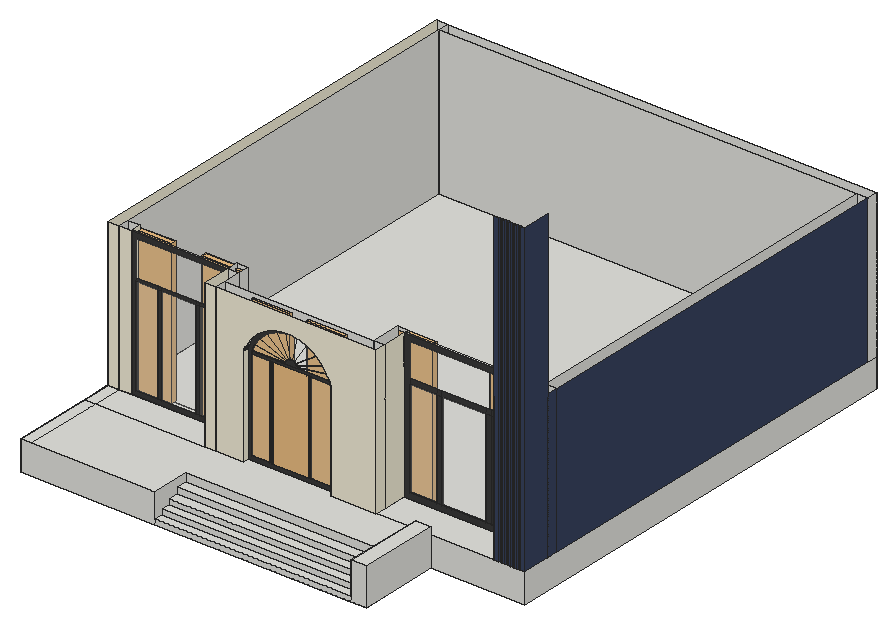
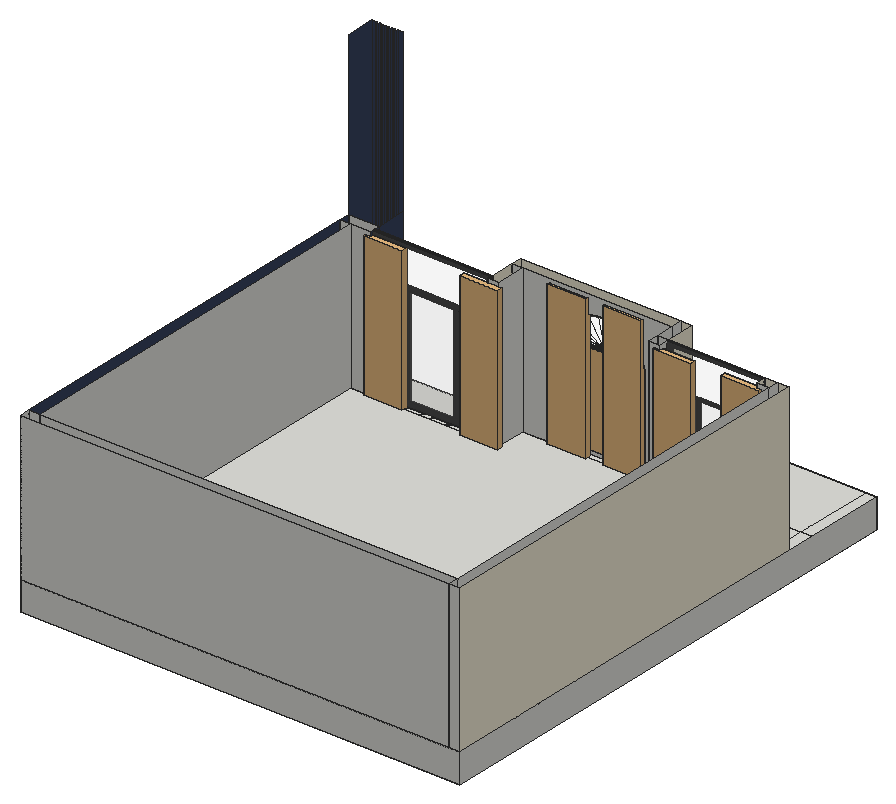
# SketchUp Ruby script. Lengths in inches.
U = 1.inch
M = Sketchup.active_model
def pt(a) = Geom::Point3d.new(a.map { |v| v * U })
def face(e, loops, mat)
  f = e.add_face(loops[0].map { |a| pt(a) })
  loops[1..].each { |l| e.add_face(l.map { |a| pt(a) }).erase! }
  f.material = f.back_material = mat if mat
  f
end
# faces: each face lists its corners as indices into pts; further lists are holes
def faces(e, pts, list, mat = nil) = list.each { |f| face(e, (f[0].is_a?(Array) ? f : [f]).map { |l| l.map { |i| pts[i] } }, mat) }
# xy, xz, yz: faces in a plane at the given z, y or x. An outline is a flat list of corners, or four numbers for a rectangle; further outlines are holes
def ring(l) = l.size == 4 ? [[l[0], l[1]], [l[2], l[1]], [l[2], l[3]], [l[0], l[3]]] : l.each_slice(2).to_a
def flat(e, list, mat, &to3) = list.each { |f| face(e, (f[0].is_a?(Array) ? f : [f]).map { |l| ring(l).map { |u, v| to3.(u, v) } }, mat) }
def xy(e, z, list, mat = nil) = flat(e, list, mat) { |x, y| [x, y, z] }
def xz(e, y, list, mat = nil) = flat(e, list, mat) { |x, z| [x, y, z] }
def yz(e, x, list, mat = nil) = flat(e, list, mat) { |y, z| [x, y, z] }
def lines(e, pts, list) = list.each { |a, b| e.add_line(pt(pts[a]), pt(pts[b])) }
# prism: a flat outline (further loops are holes) pulled along v
def prism(e, loops, v, mat = nil)
  f = face(e, loops, mat); d = Geom::Vector3d.new(v.map { |x| x * U })
  f.pushpull(f.normal.samedirection?(d) ? d.length : -d.length)
end
def box(e, o, s, mat = nil) = prism(e, [[o, [o[0] + s[0], o[1], o[2]], [o[0] + s[0], o[1] + s[1], o[2]], [o[0], o[1] + s[1], o[2]]]], [0, 0, s[2]], mat)
def at(x, y, z, deg = 0) = Geom::Transformation.translation(pt([x, y, z])) * Geom::Transformation.rotation(ORIGIN, Z_AXIS, deg.degrees)
def axes(o, x, y, z) = Geom::Transformation.new([*x, 0, *y, 0, *z, 0, *pt(o).to_a, 1])
def part(name) = M.definitions.add(name)
# library, detail: a bought-in or finely detailed component or shape, given as its bounding box
def library(name, o, s) = part(name).tap { |d| box(d.entities, o, s) }
def detail(e, o, s) = box(e.add_group.entities, o, s)
def put(e, d, t, mat = nil) = e.add_instance(d, t).tap { |i| i.material = mat if mat }
def group(e, t, mat = nil) = e.add_group.tap { |g| g.transformation = t; g.material = mat if mat }.entities
root = M.entities
M.materials.add("0360 AP 9644 Monsoon Midnight-N").color = [56, 67, 95]
M.materials.add("0905 AP 7844 MILD YELLOW").color = [242, 237, 215]
M.materials.add("Glass Clear 001").color = [246, 246, 246]
M.materials["Glass Clear 001"].alpha = 0.1
M.materials.add("[Color M07]").color = [58, 58, 58]
c1 = library("Curtains 004",[-15.59,-2.26,0],[31.18,4.52,116.91])
c2 = library("Door 243 053",[-21.6,-2.79,-0.07],[43.2,5.58,82.64])
xy(root,-24,[[24,0,24,425.9375,384,425.9375,384,65.9375,307.25,65.9375,307.25,0]])
xy(root,-19.71,[[134.39,0,294.77,6.625]])
xy(root,-15.42,[[134.39,6.625,294.77,14.1875]])
xy(root,-11.11,[[134.39,14.1875,294.77,22.4375]])
xy(root,-6.36,[[134.39,22.4375,294.77,31.5625]])
xy(root,0,[[24,0,33,65.9375],[33,0,134.39,0,134.39,31.5625,294.77,31.5625,294.77,65.9375,225.17,65.9375,225.17,70.4375,153.92,70.4375,153.92,65.9375,33,65.9375],[24,65.9375,33,89.9375],[33,65.9375,122.125,89.9375],[122.125,65.9375,153.92,65.9375,153.92,70.4375,225.17,70.4375,225.17,65.9375,262.5625,65.9375,262.5625,94.4375,358.89,94.4375,358.89,98.9375,253.5625,98.9375,253.5625,74.9375,131.125,74.9375,131.125,98.9375,43.05,98.9375,43.05,89.9375,122.125,89.9375],
  [122.125,65.9375,131.125,89.9375],[131.125,65.9375,153.92,74.9375],[225.17,65.9375,262.5625,74.9375],[262.5625,65.9375,358.89,94.4375],[358.89,65.9375,362.92,65.9375,362.92,66.75,365.27,66.75,365.27,65.9375,367.92,65.9375,367.92,66.75,370.27,66.75,370.27,65.9375,372.92,65.9375,372.92,66.75,375.27,66.75,375.27,65.9375,377.92,65.9375,377.92,66.75,380.27,66.75,380.27,65.9375,384,65.9375,384,89.9375,358.89,89.9375],
  [362.92,65.9375,365.27,66.75],[367.92,65.9375,370.27,66.75],[372.92,65.9375,375.27,66.75],[377.92,65.9375,380.27,66.75],[153.92,70.4375,225.17,70.75],
  [131.125,74.9375,253.5625,74.9375,253.5625,98.9375,375,98.9375,375,416.9375,33,416.9375,33,98.9375,131.125,98.9375],[253.5625,74.9375,262.5625,98.9375],[24,89.9375,33,425.9375],[33,89.9375,43.05,98.9375],[43.05,89.9375,122.125,91.4375],
  [122.125,89.9375,131.125,98.9375],[358.89,89.9375,384,98.9375],[43.05,91.4375,122.125,98.9375],[262.5625,94.4375,358.89,96.5625],[262.5625,96.5625,358.89,98.9375],
  [375,98.9375,384,416.9375],[33,416.9375,384,425.9375]])
xy(root,3.38,[[172.1875,70.4375,174.05,70.75],[203.54,70.4375,205.49,70.75]])
xy(root,3.38,[[157.31,70.4375,172.1875,70.75],[174.05,70.4375,203.54,70.75],[205.49,70.4375,221.79,70.75]],"[Color M07]")
xy(root,3.74,[[46.79,89.9375,64.29,90.25],[67.49,89.9375,95.54,90.25],[98.74,89.9375,118.39,90.25]],"[Color M07]")
xy(root,4.37,[[266.94,94.4375,289.69,95.5],[293.7,94.4375,329.88,95.5],[334.04,94.4375,354.52,95.5]],"[Color M07]")
xy(root,6.4375,[[294.77,0,307.25,65.9375]])
xy(root,78.21,[[157.31,70.4375,172.1875,70.75],[174.05,70.4375,203.54,70.75],[205.49,70.4375,221.79,70.75]],"[Color M07]")
xy(root,84.36,[[46.79,89.9375,64.29,90.25],[67.49,89.9375,95.54,90.25],[98.74,89.9375,118.39,90.25]])
xy(root,84.51,[[266.94,94.4375,289.69,95.5],[293.7,94.4375,329.88,95.5],[334.04,94.4375,354.52,95.5]])
xz(root,0,[[24,-24,134.39,0],[134.39,-24,294.77,-19.71],[294.77,-24,307.25,6.4375]])
xz(root,6.625,[[134.39,-19.71,294.77,-15.42]])
xz(root,14.1875,[[134.39,-15.42,294.77,-11.11]])
xz(root,22.4375,[[134.39,-11.11,294.77,-6.36]])
xz(root,31.5625,[[134.39,-6.36,294.77,0]])
xz(root,65.9375,[[307.25,-24,384,0],[294.77,0,307.25,6.4375]])
xz(root,65.9375,[[358.89,0,362.92,252],[365.27,0,367.92,252],[370.27,0,372.92,252],[375.27,0,377.92,252],[380.27,0,384,252]],"0360 AP 9644 Monsoon Midnight-N")
xz(root,65.9375,[[122.125,0,131.125,120],[131.125,0,153.92,0,153.92,81.13,154.18,81.87,154.45,82.6,154.73,83.33,155.03,84.05,155.35,84.77,155.68,85.48,156.02,86.18,156.38,86.87,156.76,87.56,157.15,88.24,157.55,88.91,157.96,89.57,158.39,90.22,158.84,90.87,159.29,91.5,159.76,92.125,160.25,92.74,160.74,93.35,161.25,93.94,161.77,94.53,162.3,95.1,162.84,95.66,163.4,96.21,163.97,96.75,164.54,97.28,165.13,97.79,165.73,98.29,166.34,98.78,166.96,99.26,167.59,99.72,168.23,100.17,168.875,100.61,169.53,101.03,170.2,101.44,170.875,101.84,171.56,102.22,172.25,102.59,172.94,102.94,173.65,103.28,174.36,103.6,175.08,103.91,175.8,104.21,176.53,104.48,177.27,104.75,178.01,105,178.76,105.23,179.51,105.45,180.26,105.65,181.02,105.83,181.79,106,182.55,106.16,183.32,106.29,184.1,106.41,184.87,106.52,185.65,106.61,186.42,106.68,187.2,106.74,187.99,106.78,188.77,106.8,189.55,106.8125,190.49,106.8,191.42,106.77,192.36,106.71,193.29,106.625,194.23,106.52,195.16,106.39,196.08,106.24,197,106.06,197.92,105.87,198.83,105.65,199.74,105.4,200.64,105.14,201.53,104.85,202.42,104.54,203.29,104.21,204.16,103.85,205.02,103.48,205.87,103.08,206.71,102.66,207.54,102.22,208.36,101.76,209.16,101.28,209.96,100.78,210.74,100.26,211.51,99.72,212.26,99.16,213,98.59,213.73,97.99,214.4375,97.38,215.13,96.75,215.81,96.1,216.47,95.4375,217.12,94.76,217.75,94.06,218.36,93.35,218.95,92.62,219.52,91.88,220.08,91.12,220.62,90.35,221.13,89.57,221.63,88.77,222.11,87.97,222.57,87.15,223,86.32,223.42,85.48,223.8125,84.625,224.18,83.76,224.54,82.89,224.87,82.02,225.17,81.13,225.17,0,262.5625,0,262.5625,120,131.125,120]],"0905 AP 7844 MILD YELLOW")
xz(root,66.75,[[362.92,0,365.27,252],[367.92,0,370.27,252],[372.92,0,375.27,252],[377.92,0,380.27,252]],"0360 AP 9644 Monsoon Midnight-N")
xz(root,70.4375,[[[153.92,0,225.17,0,225.17,81.13,224.87,82.02,224.54,82.89,224.18,83.76,223.8125,84.625,223.42,85.48,223,86.32,222.57,87.15,222.11,87.97,221.63,88.77,221.13,89.57,220.62,90.35,220.08,91.12,219.52,91.88,218.95,92.62,218.36,93.35,217.75,94.06,217.12,94.76,216.47,95.4375,215.81,96.1,215.13,96.75,214.4375,97.38,213.73,97.99,213,98.59,212.26,99.16,211.51,99.72,210.74,100.26,209.96,100.78,209.16,101.28,208.36,101.76,207.54,102.22,206.71,102.66,205.87,103.08,205.02,103.48,204.16,103.85,203.29,104.21,202.42,104.54,201.53,104.85,200.64,105.14,199.74,105.4,198.83,105.65,197.92,105.87,197,106.06,196.08,106.24,195.16,106.39,194.23,106.52,193.29,106.625,192.36,106.71,191.42,106.77,190.49,106.8,189.55,106.8125,188.77,106.8,187.99,106.78,187.2,106.74,186.42,106.68,185.65,106.61,184.87,106.52,184.1,106.41,183.32,106.29,182.55,106.16,181.79,106,181.02,105.83,180.26,105.65,179.51,105.45,178.76,105.23,178.01,105,177.27,104.75,176.53,104.48,175.8,104.21,175.08,103.91,174.36,103.6,173.65,103.28,172.94,102.94,172.25,102.59,171.56,102.22,170.875,101.84,170.2,101.44,169.53,101.03,168.875,100.61,168.23,100.17,167.59,99.72,166.96,99.26,166.34,98.78,165.73,98.29,165.13,97.79,164.54,97.28,163.97,96.75,163.4,96.21,162.84,95.66,162.3,95.1,161.77,94.53,161.25,93.94,160.74,93.35,160.25,92.74,159.76,92.125,159.29,91.5,158.84,90.87,158.39,90.22,157.96,89.57,157.55,88.91,157.15,88.24,156.76,87.56,156.38,86.87,156.02,86.18,155.68,85.48,155.35,84.77,155.03,84.05,154.73,83.33,154.45,82.6,154.18,81.87,153.92,81.13],[157.31,3.38,157.31,80.5625,157.61,81.4,157.87,82.0625,158.15,82.72,158.43,83.37,158.73,84.01,159.05,84.65,159.375,85.28,159.71,85.91,160.07,86.53,160.43,87.14,160.8125,87.74,161.2,88.33,161.6,88.92,162.02,89.5,162.45,90.07,162.89,90.625,163.34,91.18,163.8,91.72,164.27,92.25,164.76,92.77,165.25,93.28,165.76,93.78,166.27,94.27,166.8,94.75,167.33,95.22,167.88,95.68,168.43,96.12,169.57,96.98,170.15,97.39,170.74,97.78,171.34,98.17,171.94,98.54,172.56,98.9,173.18,99.25,174.44,99.91,175.08,100.21,175.73,100.51,176.38,100.79,177.04,101.06,177.71,101.31,178.375,101.55,179.05,101.78,179.73,101.99,180.41,102.18,181.1,102.37,181.79,102.54,182.49,102.69,183.18,102.83,183.88,102.96,184.59,103.07,185.29,103.16,186,103.24,186.71,103.31,187.42,103.36,188.125,103.4,188.84,103.42,189.54,103.43,190.4,103.42,191.26,103.39,192.11,103.33,192.96,103.26,193.81,103.16,194.65,103.04,195.49,102.91,196.33,102.75,197.17,102.57,198,102.37,198.82,102.15,199.64,101.9,200.45,101.64,201.26,101.36,202.06,101.06,202.85,100.73,203.63,100.39,204.4,100.03,205.16,99.65,205.92,99.25,206.66,98.83,207.4,98.4,208.12,97.94,208.83,97.47,209.53,96.98,210.21,96.47,210.89,95.94,211.55,95.4,212.19,94.85,212.83,94.27,213.44,93.68,214.05,93.08,214.63,92.46,215.2,91.82,215.76,91.18,216.3,90.51,216.82,89.84,217.33,89.15,217.82,88.45,218.29,87.74,218.74,87.02,219.17,86.28,219.59,85.54,219.99,84.78,220.36,84.01,220.72,83.24,221.0625,82.46,221.38,81.67,221.68,80.87,221.79,80.56,221.79,3.38]],[172.1875,3.38,174.05,78.21],[203.54,3.38,205.49,78.21],[157.31,78.21,221.79,78.21,221.79,80.56,195.3125,80.63,183.84,80.66,157.37,80.73,157.31,80.5625],[195.3125,80.63,194.98,81.38,194.8,81.78,194.43,82.28,194.06,82.79,193.51,83.29,193.12,83.63,192.03,84.26,191.98,84.28,190.84,84.65,190.49,84.69,189.59,84.79,188.68,84.69,188.34,84.66,187.3125,84.33,187.14,84.28,186.05,83.65,185.97,83.59,185.11,82.82,184.97,82.625,184.36,81.81,184.26,81.58,183.84,80.66]],"[Color M07]")
xz(root,70.75,[[[153.92,0,153.92,81.13,154.18,81.87,154.45,82.6,154.73,83.33,155.03,84.05,155.35,84.77,155.68,85.48,156.02,86.18,156.38,86.87,156.76,87.56,157.15,88.24,157.55,88.91,157.96,89.57,158.39,90.22,158.84,90.87,159.29,91.5,159.76,92.125,160.25,92.74,160.74,93.35,161.25,93.94,161.77,94.53,162.3,95.1,162.84,95.66,163.4,96.21,163.97,96.75,164.54,97.28,165.13,97.79,165.73,98.29,166.34,98.78,166.96,99.26,167.59,99.72,168.23,100.17,168.875,100.61,169.53,101.03,170.2,101.44,170.875,101.84,171.56,102.22,172.25,102.59,172.94,102.94,173.65,103.28,174.36,103.6,175.08,103.91,175.8,104.21,176.53,104.48,177.27,104.75,178.01,105,178.76,105.23,179.51,105.45,180.26,105.65,181.02,105.83,181.79,106,182.55,106.16,183.32,106.29,184.1,106.41,184.87,106.52,185.65,106.61,186.42,106.68,187.2,106.74,187.99,106.78,188.77,106.8,189.55,106.8125,190.49,106.8,191.42,106.77,192.36,106.71,193.29,106.625,194.23,106.52,195.16,106.39,196.08,106.24,197,106.06,197.92,105.87,198.83,105.65,199.74,105.4,200.64,105.14,201.53,104.85,202.42,104.54,203.29,104.21,204.16,103.85,205.02,103.48,205.87,103.08,206.71,102.66,207.54,102.22,208.36,101.76,209.16,101.28,209.96,100.78,210.74,100.26,211.51,99.72,212.26,99.16,213,98.59,213.73,97.99,214.4375,97.38,215.13,96.75,215.81,96.1,216.47,95.4375,217.12,94.76,217.75,94.06,218.36,93.35,218.95,92.62,219.52,91.88,220.08,91.12,220.62,90.35,221.13,89.57,221.63,88.77,222.11,87.97,222.57,87.15,223,86.32,223.42,85.48,223.8125,84.625,224.18,83.76,224.54,82.89,224.87,82.02,225.17,81.13,225.17,0],[157.31,3.38,221.79,3.38,221.79,80.56,221.68,80.87,221.38,81.67,221.0625,82.46,220.72,83.24,220.36,84.01,219.99,84.78,219.59,85.54,219.17,86.28,218.74,87.02,218.29,87.74,217.82,88.45,217.33,89.15,216.82,89.84,216.3,90.51,215.76,91.18,215.2,91.82,214.63,92.46,214.05,93.08,213.44,93.68,212.83,94.27,212.19,94.85,211.55,95.4,210.89,95.94,210.21,96.47,209.53,96.98,208.83,97.47,208.12,97.94,207.4,98.4,206.66,98.83,205.92,99.25,205.16,99.65,204.4,100.03,203.63,100.39,202.85,100.73,202.06,101.06,201.26,101.36,200.45,101.64,199.64,101.9,198.82,102.15,198,102.37,197.17,102.57,196.33,102.75,195.49,102.91,194.65,103.04,193.81,103.16,192.96,103.26,192.11,103.33,191.26,103.39,190.4,103.42,189.54,103.43,188.84,103.42,188.125,103.4,187.42,103.36,186.71,103.31,186,103.24,185.29,103.16,184.59,103.07,183.88,102.96,183.18,102.83,182.49,102.69,181.79,102.54,181.1,102.37,180.41,102.18,179.73,101.99,179.05,101.78,178.375,101.55,177.71,101.31,177.04,101.06,176.38,100.79,175.73,100.51,175.08,100.21,174.44,99.91,173.18,99.25,172.56,98.9,171.94,98.54,171.34,98.17,170.74,97.78,170.15,97.39,169.57,96.98,168.43,96.12,167.88,95.68,167.33,95.22,166.8,94.75,166.27,94.27,165.76,93.78,165.25,93.28,164.76,92.77,164.27,92.25,163.8,91.72,163.34,91.18,162.89,90.625,162.45,90.07,162.02,89.5,161.6,88.92,161.2,88.33,160.8125,87.74,160.43,87.14,160.07,86.53,159.71,85.91,159.375,85.28,159.05,84.65,158.73,84.01,158.43,83.37,158.15,82.72,157.87,82.0625,157.61,81.4,157.31,80.5625]]])
xz(root,70.75,[[157.31,3.38,172.1875,78.21],[205.49,3.38,221.79,78.21],[221.79,80.56,221.68,80.87,221.38,81.67,221.0625,82.46,220.72,83.24,220.36,84.01,219.99,84.78,194.98,81.38,195.3125,80.63],[183.84,80.66,184.26,81.58,159.71,85.91,159.375,85.28,159.05,84.65,158.73,84.01,158.43,83.37,158.15,82.72,157.87,82.0625,157.61,81.4,157.37,80.73],[194.98,81.38,219.99,84.78,219.59,85.54,219.17,86.28,218.74,87.02,218.29,87.74,217.82,88.45,217.33,89.15,216.82,89.84,194.43,82.28,194.8,81.78],
  [184.26,81.58,184.36,81.81,184.97,82.625,163.8,91.72,163.34,91.18,162.89,90.625,162.45,90.07,162.02,89.5,161.6,88.92,161.2,88.33,160.8125,87.74,160.43,87.14,160.07,86.53,159.71,85.91],[194.43,82.28,216.82,89.84,216.3,90.51,215.76,91.18,215.2,91.82,214.63,92.46,214.05,93.08,213.44,93.68,212.83,94.27,212.19,94.85,211.55,95.4,193.51,83.29,194.06,82.79],[184.97,82.625,185.11,82.82,185.97,83.59,169.57,96.98,168.43,96.12,167.88,95.68,167.33,95.22,166.8,94.75,166.27,94.27,165.76,93.78,165.25,93.28,164.76,92.77,164.27,92.25,163.8,91.72],[193.51,83.29,211.55,95.4,210.89,95.94,210.21,96.47,209.53,96.98,208.83,97.47,208.12,97.94,207.4,98.4,206.66,98.83,205.92,99.25,205.16,99.65,204.4,100.03,203.63,100.39,202.85,100.73,191.98,84.28,192.03,84.26,193.12,83.63],[185.97,83.59,186.05,83.65,187.14,84.28,187.3125,84.33,177.04,101.06,176.38,100.79,175.73,100.51,175.08,100.21,174.44,99.91,173.18,99.25,172.56,98.9,171.94,98.54,171.34,98.17,170.74,97.78,170.15,97.39,169.57,96.98],
  [191.98,84.28,202.85,100.73,202.06,101.06,201.26,101.36,200.45,101.64,199.64,101.9,198.82,102.15,198,102.37,197.17,102.57,196.33,102.75,195.49,102.91,194.65,103.04,190.49,84.69,190.84,84.65],[187.3125,84.33,188.34,84.66,188.68,84.69,184.59,103.07,183.88,102.96,183.18,102.83,182.49,102.69,181.79,102.54,181.1,102.37,180.41,102.18,179.73,101.99,179.05,101.78,178.375,101.55,177.71,101.31,177.04,101.06],[188.68,84.69,189.59,84.79,190.49,84.69,194.65,103.04,193.81,103.16,192.96,103.26,192.11,103.33,191.26,103.39,190.4,103.42,189.54,103.43,188.84,103.42,188.125,103.4,187.42,103.36,186.71,103.31,186,103.24,185.29,103.16,184.59,103.07]],"Glass Clear 001")
xz(root,74.9375,[[131.125,0,131.125,120,253.5625,120,253.5625,0,225.17,0,225.17,81.13,224.87,82.02,224.54,82.89,224.18,83.76,223.8125,84.625,223.42,85.48,223,86.32,222.57,87.15,222.11,87.97,221.63,88.77,221.13,89.57,220.62,90.35,220.08,91.12,219.52,91.88,218.95,92.62,218.36,93.35,217.75,94.06,217.12,94.76,216.47,95.4375,215.81,96.1,215.13,96.75,214.4375,97.38,213.73,97.99,213,98.59,212.26,99.16,211.51,99.72,210.74,100.26,209.96,100.78,209.16,101.28,208.36,101.76,207.54,102.22,206.71,102.66,205.87,103.08,205.02,103.48,204.16,103.85,203.29,104.21,202.42,104.54,201.53,104.85,200.64,105.14,199.74,105.4,198.83,105.65,197.92,105.87,197,106.06,196.08,106.24,195.16,106.39,194.23,106.52,193.29,106.625,192.36,106.71,191.42,106.77,190.49,106.8,189.55,106.8125,188.77,106.8,187.99,106.78,187.2,106.74,186.42,106.68,185.65,106.61,184.87,106.52,184.1,106.41,183.32,106.29,182.55,106.16,181.79,106,181.02,105.83,180.26,105.65,179.51,105.45,178.76,105.23,178.01,105,177.27,104.75,176.53,104.48,175.8,104.21,175.08,103.91,174.36,103.6,173.65,103.28,172.94,102.94,172.25,102.59,171.56,102.22,170.875,101.84,170.2,101.44,169.53,101.03,168.875,100.61,168.23,100.17,167.59,99.72,166.96,99.26,166.34,98.78,165.73,98.29,165.13,97.79,164.54,97.28,163.97,96.75,163.4,96.21,162.84,95.66,162.3,95.1,161.77,94.53,161.25,93.94,160.74,93.35,160.25,92.74,159.76,92.125,159.29,91.5,158.84,90.87,158.39,90.22,157.96,89.57,157.55,88.91,157.15,88.24,156.76,87.56,156.38,86.87,156.02,86.18,155.68,85.48,155.35,84.77,155.03,84.05,154.73,83.33,154.45,82.6,154.18,81.87,153.92,81.13,153.92,0],[253.5625,0,262.5625,120]])
xz(root,89.9375,[[122.125,0,131.125,120],[358.89,0,384,120]])
xz(root,89.9375,[[24,0,33,120],[33,0,43.05,120]],"0905 AP 7844 MILD YELLOW")
xz(root,89.9375,[[[43.05,0,122.125,120],[46.79,3.74,118.39,116.26]],[64.29,3.74,67.49,84.36],[95.54,3.74,98.74,84.36],[46.79,84.36,64.29,86.69],[64.29,84.36,67.49,86.69],
  [67.49,84.36,95.54,86.69],[95.54,84.36,98.74,86.69],[98.74,84.36,118.39,86.69]],"[Color M07]")
xz(root,90.25,[[46.79,3.74,64.29,84.36],[67.49,3.74,95.54,84.36],[98.74,3.74,118.39,84.36]],"Glass Clear 001")
xz(root,91.4375,[[43.05,0,122.125,120]],"Glass Clear 001")
xz(root,94.4375,[[[262.5625,0,358.89,120],[266.94,4.37,354.52,115.63]],[289.69,4.37,293.7,84.51],[329.88,4.37,334.04,84.51],[266.94,84.51,289.69,88.49],[289.69,84.51,293.7,88.49],
  [293.7,84.51,329.88,88.49],[329.88,84.51,334.04,88.49],[334.04,84.51,354.52,88.49]],"[Color M07]")
xz(root,95.5,[[266.94,4.37,289.69,84.51],[293.7,4.37,329.88,84.51],[334.04,4.37,354.52,84.51]],"Glass Clear 001")
xz(root,96.5625,[[262.5625,0,358.89,120]],"Glass Clear 001")
xz(root,98.9375,[[33,0,43.05,120],[122.125,0,131.125,120],[253.5625,0,262.5625,120],[358.89,0,375,120],[375,0,384,120]])
xz(root,416.9375,[[33,0,375,120],[375,0,384,120]])
xz(root,425.9375,[[24,-24,384,0],[24,0,33,120],[33,0,384,120]])
yz(root,24,[[0,-24,425.9375,0]])
yz(root,24,[[89.9375,0,425.9375,120]],"0905 AP 7844 MILD YELLOW")
yz(root,33,[[89.9375,0,98.9375,120],[98.9375,0,416.9375,120],[416.9375,0,425.9375,120]])
yz(root,43.05,[[91.4375,0,98.9375,120]],"0905 AP 7844 MILD YELLOW")
yz(root,43.05,[[89.9375,0,91.4375,120]],"[Color M07]")
yz(root,46.79,[[89.9375,3.74,90.25,84.36]],"[Color M07]")
yz(root,64.29,[[89.9375,3.74,90.25,84.36]],"[Color M07]")
yz(root,67.49,[[89.9375,3.74,90.25,84.36]],"[Color M07]")
yz(root,95.54,[[89.9375,3.74,90.25,84.36]],"[Color M07]")
yz(root,98.74,[[89.9375,3.74,90.25,84.36]],"[Color M07]")
yz(root,118.39,[[89.9375,3.74,90.25,84.36]],"[Color M07]")
yz(root,122.125,[[91.4375,0,98.9375,120]])
yz(root,122.125,[[65.9375,0,89.9375,120]],"0905 AP 7844 MILD YELLOW")
yz(root,122.125,[[89.9375,0,91.4375,120]],"[Color M07]")
yz(root,131.125,[[65.9375,0,74.9375,120],[74.9375,0,89.9375,120],[89.9375,0,98.9375,120]])
yz(root,134.39,[[0,-19.71,6.625,-19.71,6.625,-15.42,14.1875,-15.42,14.1875,-11.11,22.4375,-11.11,22.4375,-6.36,31.5625,-6.36,31.5625,0,0,0]])
yz(root,153.92,[[65.9375,0,70.4375,81.13],[70.75,0,74.9375,81.13]],"0905 AP 7844 MILD YELLOW")
yz(root,153.92,[[70.4375,0,70.75,81.13]],"[Color M07]")
yz(root,157.31,[[70.4375,78.21,70.75,80.5625]])
yz(root,157.31,[[70.4375,3.38,70.75,78.21]],"[Color M07]")
yz(root,172.1875,[[70.4375,3.38,70.75,78.21]],"[Color M07]")
yz(root,174.05,[[70.4375,3.38,70.75,78.21]],"[Color M07]")
yz(root,203.54,[[70.4375,3.38,70.75,78.21]],"[Color M07]")
yz(root,205.49,[[70.4375,3.38,70.75,78.21]],"[Color M07]")
yz(root,221.79,[[70.4375,78.21,70.75,80.56]])
yz(root,221.79,[[70.4375,3.38,70.75,78.21]],"[Color M07]")
yz(root,225.17,[[65.9375,0,70.4375,81.13],[70.75,0,74.9375,81.13]],"0905 AP 7844 MILD YELLOW")
yz(root,225.17,[[70.4375,0,70.75,81.13]],"[Color M07]")
yz(root,253.5625,[[74.9375,0,98.9375,120]])
yz(root,262.5625,[[65.9375,0,74.9375,120],[74.9375,0,94.4375,120],[96.5625,0,98.9375,120]],"0905 AP 7844 MILD YELLOW")
yz(root,262.5625,[[94.4375,0,96.5625,120]],"[Color M07]")
yz(root,266.94,[[94.4375,4.37,95.5,84.51]],"[Color M07]")
yz(root,289.69,[[94.4375,4.37,95.5,84.51]],"[Color M07]")
yz(root,293.7,[[94.4375,4.37,95.5,84.51]],"[Color M07]")
yz(root,294.77,[[0,-19.71,0,6.4375,65.9375,6.4375,65.9375,0,31.5625,0,31.5625,-6.36,22.4375,-6.36,22.4375,-11.11,14.1875,-11.11,14.1875,-15.42,6.625,-15.42,6.625,-19.71]])
yz(root,307.25,[[0,-24,65.9375,6.4375]])
yz(root,329.88,[[94.4375,4.37,95.5,84.51]],"[Color M07]")
yz(root,334.04,[[94.4375,4.37,95.5,84.51]],"[Color M07]")
yz(root,354.52,[[94.4375,4.37,95.5,84.51]],"[Color M07]")
yz(root,358.89,[[65.9375,0,89.9375,120],[89.9375,0,94.4375,120],[96.5625,0,98.9375,120]],"0360 AP 9644 Monsoon Midnight-N")
yz(root,358.89,[[94.4375,0,96.5625,120]],"[Color M07]")
yz(root,362.92,[[65.9375,0,66.75,252]],"0360 AP 9644 Monsoon Midnight-N")
yz(root,365.27,[[65.9375,0,66.75,252]],"0360 AP 9644 Monsoon Midnight-N")
yz(root,367.92,[[65.9375,0,66.75,252]],"0360 AP 9644 Monsoon Midnight-N")
yz(root,370.27,[[65.9375,0,66.75,252]],"0360 AP 9644 Monsoon Midnight-N")
yz(root,372.92,[[65.9375,0,66.75,252]],"0360 AP 9644 Monsoon Midnight-N")
yz(root,375,[[98.9375,0,416.9375,120]])
yz(root,375.27,[[65.9375,0,66.75,252]],"0360 AP 9644 Monsoon Midnight-N")
yz(root,377.92,[[65.9375,0,66.75,252]],"0360 AP 9644 Monsoon Midnight-N")
yz(root,380.27,[[65.9375,0,66.75,252]],"0360 AP 9644 Monsoon Midnight-N")
yz(root,384,[[65.9375,-24,425.9375,0],[416.9375,0,425.9375,120]])
yz(root,384,[[65.9375,0,89.9375,252],[89.9375,0,98.9375,120],[98.9375,0,416.9375,120]],"0360 AP 9644 Monsoon Midnight-N")
p = [[157.31,70.75,80.5625],[157.37,70.75,80.73],[157.37,70.4375,80.73],[157.31,70.4375,80.5625],[195.3125,70.75,80.63],[194.98,70.75,81.38],
  [194.98,70.4375,81.38],[195.3125,70.4375,80.63],[221.79,70.75,80.56],[221.79,70.4375,80.56],[221.68,70.75,80.87],[221.68,70.4375,80.87],
  [183.84,70.75,80.66],[183.84,70.4375,80.66],[157.61,70.75,81.4],[157.61,70.4375,81.4],[184.26,70.75,81.58],[184.26,70.4375,81.58],
  [221.38,70.75,81.67],[221.38,70.4375,81.67],[153.92,65.9375,81.13],[153.92,70.4375,81.13],[154.18,70.4375,81.87],[154.18,65.9375,81.87],
  [224.87,65.9375,82.02],[224.87,70.4375,82.02],[225.17,70.4375,81.13],[225.17,65.9375,81.13],[154.18,70.75,81.87],[153.92,70.75,81.13],
  [225.17,70.75,81.13],[224.87,70.75,82.02],[154.18,74.9375,81.87],[153.92,74.9375,81.13],[225.17,74.9375,81.13],[224.87,74.9375,82.02],
  [157.87,70.75,82.0625],[157.87,70.4375,82.0625],[194.8,70.75,81.78],[194.8,70.4375,81.78],[184.36,70.75,81.81],[184.36,70.4375,81.81],
  [221.0625,70.75,82.46],[221.0625,70.4375,82.46],[184.97,70.75,82.625],[184.97,70.4375,82.625],[194.43,70.75,82.28],[194.43,70.4375,82.28],
  [154.45,70.4375,82.6],[154.45,65.9375,82.6],[154.45,70.75,82.6],[154.45,74.9375,82.6],[224.54,65.9375,82.89],[224.54,70.4375,82.89],
  [224.54,70.75,82.89],[224.54,74.9375,82.89],[158.15,70.75,82.72],[158.15,70.4375,82.72],[194.06,70.75,82.79],[194.06,70.4375,82.79],
  [220.72,70.75,83.24],[220.72,70.4375,83.24],[154.73,70.4375,83.33],[154.73,65.9375,83.33],[154.73,70.75,83.33],[185.11,70.75,82.82],
  [185.11,70.4375,82.82],[154.73,74.9375,83.33],[158.43,70.75,83.37],[158.43,70.4375,83.37],[185.97,70.75,83.59],[185.97,70.4375,83.59],
  [193.51,70.75,83.29],[193.51,70.4375,83.29],[224.18,65.9375,83.76],[224.18,70.4375,83.76],[224.18,70.75,83.76],[224.18,74.9375,83.76],
  [220.36,70.75,84.01],[220.36,70.4375,84.01],[155.03,70.4375,84.05],[155.03,65.9375,84.05],[155.03,70.75,84.05],[193.12,70.75,83.63],
  [193.12,70.4375,83.63],[155.03,74.9375,84.05],[158.73,70.75,84.01],[158.73,70.4375,84.01],[186.05,70.75,83.65],[186.05,70.4375,83.65],
  [192.03,70.75,84.26],[192.03,70.4375,84.26],[187.14,70.75,84.28],[187.14,70.4375,84.28],[223.8125,65.9375,84.625],[223.8125,70.4375,84.625],
  [223.8125,70.75,84.625],[223.8125,74.9375,84.625],[159.05,70.75,84.65],[159.05,70.4375,84.65],[219.99,70.75,84.78],[219.99,70.4375,84.78],
  [155.35,70.4375,84.77],[155.35,65.9375,84.77],[155.35,70.75,84.77],[155.35,74.9375,84.77],[187.3125,70.75,84.33],[187.3125,70.4375,84.33],
  [188.34,70.75,84.66],[188.34,70.4375,84.66],[191.98,70.75,84.28],[190.84,70.75,84.65],[190.84,70.4375,84.65],[191.98,70.4375,84.28],
  [223.42,65.9375,85.48],[223.42,70.4375,85.48],[223.42,70.75,85.48],[223.42,74.9375,85.48],[159.375,70.75,85.28],[159.375,70.4375,85.28],
  [188.68,70.75,84.69],[188.68,70.4375,84.69],[189.59,70.75,84.79],[189.59,70.4375,84.79],[190.49,70.75,84.69],[190.49,70.4375,84.69],
  [155.68,70.4375,85.48],[155.68,65.9375,85.48],[155.68,70.75,85.48],[219.59,70.75,85.54],[219.59,70.4375,85.54],[155.68,74.9375,85.48]]
faces(root,p,[[0,1,2,3]])
faces(root,p,[[4,5,6,7],[8,4,7,9],[10,8,9,11],[12,1,2,13],[1,14,15,2],[16,12,13,17],[18,10,11,19],[28,29,21,22],
  [30,31,25,26],[14,36,37,15],[5,38,39,6],[40,16,17,41],[42,18,19,43],[44,40,41,45],[38,46,47,39],[50,28,22,48],
  [31,54,53,25],[36,56,57,37],[46,58,59,47],[60,42,43,61],[64,50,48,62],[65,44,45,66],[56,68,69,57],[70,65,66,71],
  [58,72,73,59],[54,76,75,53],[78,60,61,79],[82,64,62,80],[72,83,84,73],[68,86,87,69],[88,70,71,89],[83,90,91,84],
  [92,88,89,93],[76,96,95,75],[86,98,99,87],[100,78,79,101],[104,82,80,102],[106,92,93,107],[108,106,107,109],[110,111,112,113],
  [90,110,113,91],[96,116,115,95],[98,118,119,99],[120,108,109,121],[122,120,121,123],[124,122,123,125],[111,124,125,112],[128,104,102,126],
  [129,100,101,130]],"[Color M07]")
faces(root,p,[[20,21,22,23],[24,25,26,27],[32,28,29,33],[34,30,31,35],[23,22,48,49],[51,50,28,32],[52,53,25,24],[35,31,54,55],
  [49,48,62,63],[67,64,50,51],[74,75,53,52],[55,54,76,77],[63,62,80,81],[85,82,64,67],[94,95,75,74],[77,76,96,97],
  [81,80,102,103],[105,104,82,85],[114,115,95,94],[97,96,116,117],[103,102,126,127],[131,128,104,105]],"0905 AP 7844 MILD YELLOW")
put(root,c1,at(346.95,98.9375,0))
put(root,c1,at(266.78,101.15,0))
put(root,c1,at(55.0625,98.9375,0))
put(root,c1,at(110.81,98.9375,0))
put(root,c1,at(170.73,74.9375,0))
put(root,c1,at(215.99,74.9375,0))
put(root,c2,axes([188.76,70.6,3.4],[-0.68671,0,0],[0,-0.07263,0],[0,0,0.90613]))
